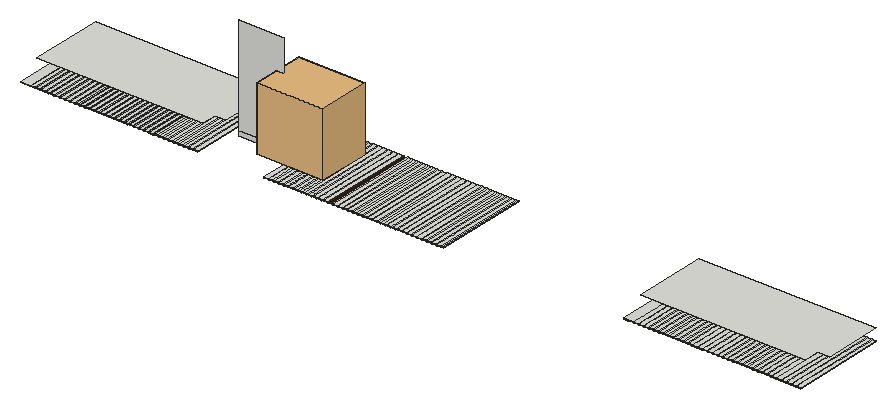
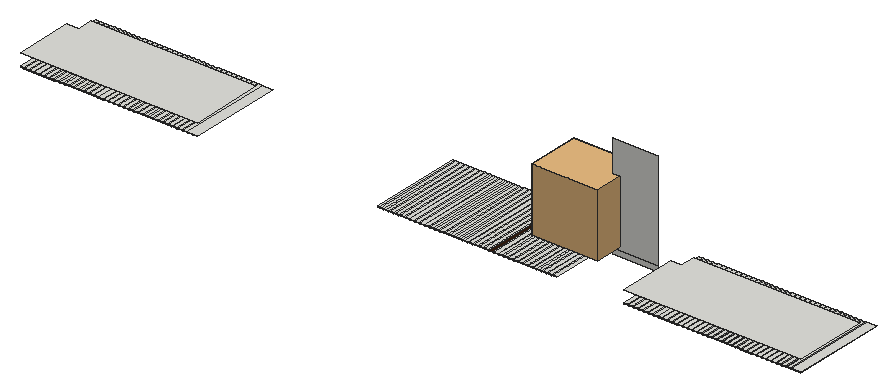
# SketchUp Ruby script. Lengths in inches.
U = 1.inch
M = Sketchup.active_model
def pt(a) = Geom::Point3d.new(a.map { |v| v * U })
def face(e, loops, mat)
  f = e.add_face(loops[0].map { |a| pt(a) })
  loops[1..].each { |l| e.add_face(l.map { |a| pt(a) }).erase! }
  f.material = f.back_material = mat if mat
  f
end
# faces: each face lists its corners as indices into pts; further lists are holes
def faces(e, pts, list, mat = nil) = list.each { |f| face(e, (f[0].is_a?(Array) ? f : [f]).map { |l| l.map { |i| pts[i] } }, mat) }
# xy, xz, yz: faces in a plane at the given z, y or x. An outline is a flat list of corners, or four numbers for a rectangle; further outlines are holes
def ring(l) = l.size == 4 ? [[l[0], l[1]], [l[2], l[1]], [l[2], l[3]], [l[0], l[3]]] : l.each_slice(2).to_a
def flat(e, list, mat, &to3) = list.each { |f| face(e, (f[0].is_a?(Array) ? f : [f]).map { |l| ring(l).map { |u, v| to3.(u, v) } }, mat) }
def xy(e, z, list, mat = nil) = flat(e, list, mat) { |x, y| [x, y, z] }
def xz(e, y, list, mat = nil) = flat(e, list, mat) { |x, z| [x, y, z] }
def yz(e, x, list, mat = nil) = flat(e, list, mat) { |y, z| [x, y, z] }
def lines(e, pts, list) = list.each { |a, b| e.add_line(pt(pts[a]), pt(pts[b])) }
# prism: a flat outline (further loops are holes) pulled along v
def prism(e, loops, v, mat = nil)
  f = face(e, loops, mat); d = Geom::Vector3d.new(v.map { |x| x * U })
  f.pushpull(f.normal.samedirection?(d) ? d.length : -d.length)
end
def box(e, o, s, mat = nil) = prism(e, [[o, [o[0] + s[0], o[1], o[2]], [o[0] + s[0], o[1] + s[1], o[2]], [o[0], o[1] + s[1], o[2]]]], [0, 0, s[2]], mat)
def at(x, y, z, deg = 0) = Geom::Transformation.translation(pt([x, y, z])) * Geom::Transformation.rotation(ORIGIN, Z_AXIS, deg.degrees)
def axes(o, x, y, z) = Geom::Transformation.new([*x, 0, *y, 0, *z, 0, *pt(o).to_a, 1])
def part(name) = M.definitions.add(name)
# library, detail: a bought-in or finely detailed component or shape, given as its bounding box
def library(name, o, s) = part(name).tap { |d| box(d.entities, o, s) }
def detail(e, o, s) = box(e.add_group.entities, o, s)
def put(e, d, t, mat = nil) = e.add_instance(d, t).tap { |i| i.material = mat if mat }
def group(e, t, mat = nil) = e.add_group.tap { |g| g.transformation = t; g.material = mat if mat }.entities
root = M.entities
M.materials.add("[Wood Veneer 01]").color = [51, 28, 15]
c1 = library("Round Planter with Plant",[-35.48,-39.77,0],[80.62,63.55,77.875])
xy(root,253.5625,[[256.68,246.64,261.43,361.27],[262.68,246.64,267.43,361.27],[268.68,246.64,273.43,361.27],[274.68,246.64,279.43,361.27],[280.68,246.64,285.43,361.27],
  [286.68,246.64,291.43,361.27],[292.68,246.64,297.43,361.27],[298.68,246.64,303.43,361.27],[304.68,246.64,309.43,361.27],[310.68,246.64,315.43,361.27],
  [990.25,246.64,995,361.27],[996.25,246.64,1001,361.27],[1002.25,246.64,1007,361.27],[1008.25,246.64,1013,361.27],[1014.25,246.64,1019,361.27],
  [1020.25,246.64,1025,361.27],[1026.25,246.64,1031,361.27],[1032.25,246.64,1037,361.27],[1038.25,246.64,1043,361.27],[1044.25,246.64,1049,361.27]],"[Wood Veneer 01]")
xy(root,253.875,[[244.68,246.64,249.43,361.27],[250.68,246.64,255.43,361.27],[978.25,246.64,983,361.27],[984.25,246.64,989,361.27]],"[Wood Veneer 01]")
xy(root,253.9375,[[100.68,246.64,105.43,361.27],[106.68,246.64,111.43,361.27],[112.68,246.64,117.43,361.27],[118.68,246.64,123.43,361.27],[124.68,246.64,129.43,361.27],
  [130.68,246.64,135.43,361.27],[136.68,246.64,141.43,361.27],[142.68,246.64,147.43,361.27],[148.68,246.64,153.43,361.27],[154.68,246.64,159.43,361.27],
  [160.68,246.64,165.43,361.27],[166.68,246.64,171.43,361.27],[172.68,246.64,177.43,361.27],[178.68,246.64,183.43,361.27],[184.68,246.64,189.43,361.27],
  [190.68,246.64,195.43,361.27],[196.68,246.64,201.43,361.27],[202.68,246.64,207.43,361.27],[208.68,246.64,213.43,361.27],[214.68,246.64,219.43,361.27],
  [220.68,246.64,225.43,361.27],[226.68,246.64,231.43,361.27],[232.68,246.64,237.43,361.27],[238.68,246.64,243.43,361.27],[396.57,246.64,400.96,361.27],
  [402.57,246.64,406.96,361.27],[408.57,246.64,412.96,361.27],[414.57,246.64,418.96,361.27],[420.57,246.64,424.96,361.27],[426.57,246.64,430.96,361.27],
  [432.57,246.64,436.96,361.27],[438.57,246.64,442.96,361.27],[444.57,246.64,448.96,361.27],[450.57,246.64,454.96,361.27],[456.57,246.64,460.96,361.27],
  [462.57,246.64,466.96,361.27],[468.57,246.64,472.96,361.27],[474.57,246.64,478.96,361.27],[480.57,246.64,484.96,361.27],[486.57,246.64,490.96,361.27],
  [492.57,246.64,496.96,361.27],[498.57,246.64,502.96,361.27],[504.57,246.64,508.96,361.27],[510.57,246.64,514.96,361.27],[516.57,246.64,520.96,361.27],
  [522.57,246.64,526.96,361.27],[528.57,246.64,532.96,361.27],[534.57,246.64,538.96,361.27],[540.57,246.64,544.96,361.27],[546.57,246.64,550.96,361.27],
  [552.57,246.64,556.96,361.27],[558.57,246.64,562.96,361.27],[564.57,246.64,568.96,361.27],[570.57,246.64,574.96,361.27],[576.57,246.64,580.96,361.27],
  [582.57,246.64,586.96,361.27],[588.57,246.64,592.96,361.27],[594.57,246.64,598.96,361.27],[600.57,246.64,604.96,361.27],[606.57,246.64,610.96,361.27],
  [612.57,246.64,614.76,361.27],[834.25,246.64,839,361.27],[840.25,246.64,845,361.27],[846.25,246.64,851,361.27],[852.25,246.64,857,361.27],
  [858.25,246.64,863,361.27],[864.25,246.64,869,361.27],[870.25,246.64,875,361.27],[876.25,246.64,881,361.27],[882.25,246.64,887,361.27],
  [888.25,246.64,893,361.27],[894.25,246.64,899,361.27],[900.25,246.64,905,361.27],[906.25,246.64,911,361.27],[912.25,246.64,917,361.27],
  [918.25,246.64,923,361.27],[924.25,246.64,929,361.27],[930.25,246.64,935,361.27],[936.25,246.64,941,361.27],[942.25,246.64,947,361.27],
  [948.25,246.64,953,361.27],[954.25,246.64,959,361.27],[960.25,246.64,965,361.27],[966.25,246.64,971,361.27],[972.25,246.64,977,361.27]],"[Wood Veneer 01]")
xy(root,254.625,[[244.68,246.64,249.43,361.27],[978.25,246.64,983,361.27]])
xy(root,254.6875,[[100.18,246.64,112.68,361.27],[112.68,246.64,117.43,361.27],[117.43,246.64,118.68,361.27],[118.68,246.64,123.43,361.27],[123.43,246.64,124.68,361.27],
  [124.68,246.64,129.43,361.27],[129.43,246.64,130.68,361.27],[130.68,246.64,135.43,361.27],[135.43,246.64,136.68,361.27],[136.68,246.64,141.43,361.27],
  [141.43,246.64,142.68,361.27],[142.68,246.64,147.43,361.27],[147.43,246.64,148.68,361.27],[148.68,246.64,153.43,361.27],[153.43,246.64,154.68,361.27],
  [154.68,246.64,159.43,361.27],[159.43,246.64,160.68,361.27],[160.68,246.64,165.43,361.27],[165.43,246.64,166.68,361.27],[166.68,246.64,171.43,361.27],
  [171.43,246.64,172.68,361.27],[172.68,246.64,177.43,361.27],[177.43,246.64,178.68,361.27],[178.68,246.64,183.43,361.27],[183.43,246.64,184.68,361.27],
  [184.68,246.64,189.43,361.27],[189.43,246.64,190.68,361.27],[190.68,246.64,195.43,361.27],[195.43,246.64,196.68,361.27],[196.68,246.64,201.43,361.27],
  [201.43,246.64,202.68,361.27],[202.68,246.64,207.43,361.27],[207.43,246.64,208.68,361.27],[208.68,246.64,213.43,361.27],[213.43,246.64,214.68,361.27],
  [214.68,246.64,219.43,361.27],[219.43,246.64,220.68,361.27],[220.68,246.64,225.43,361.27],[225.43,246.64,226.68,361.27],[226.68,246.64,231.43,361.27],
  [231.43,246.64,232.68,361.27],[232.68,246.64,237.43,361.27],[237.43,246.64,238.68,361.27],[238.68,246.64,243.43,361.27],[243.43,246.64,244.68,361.27],
  [244.68,246.64,249.43,361.27],[249.43,246.64,250.68,361.27],[250.68,246.64,255.43,361.27],[255.43,246.64,256.68,361.27],[256.68,246.64,261.43,361.27],
  [261.43,246.64,262.68,361.27],[262.68,246.64,267.43,361.27],[267.43,246.64,268.68,361.27],[268.68,246.64,273.43,361.27],[273.43,246.64,274.68,361.27],
  [274.68,246.64,279.43,361.27],[279.43,246.64,280.68,361.27],[280.68,246.64,285.43,361.27],[285.43,246.64,286.68,361.27],[286.68,246.64,291.43,361.27],
  [291.43,246.64,292.68,361.27],[292.68,246.64,297.43,361.27],[297.43,246.64,298.68,361.27],[298.68,246.64,303.43,361.27],[303.43,246.64,304.68,361.27],
  [304.68,246.64,309.43,361.27],[309.43,246.64,310.68,361.27],[310.68,246.64,315.43,361.27],[396.57,246.64,400.96,361.27],[400.96,246.64,402.57,361.27],
  [402.57,246.64,406.96,361.27],[406.96,246.64,408.57,361.27],[408.57,246.64,412.96,361.27],[412.96,246.64,414.57,361.27],[414.57,246.64,418.96,361.27],
  [418.96,246.64,420.57,361.27],[420.57,246.64,424.96,361.27],[424.96,246.64,426.57,361.27],[426.57,246.64,430.96,361.27],[430.96,246.64,432.57,361.27],
  [432.57,246.64,436.96,361.27],[436.96,246.64,438.57,361.27],[438.57,246.64,442.96,361.27],[442.96,246.64,444.57,361.27],[444.57,246.64,448.96,361.27],
  [448.96,246.64,450.57,361.27],[450.57,246.64,454.96,361.27],[454.96,246.64,456.57,361.27],[456.57,246.64,460.96,361.27],[460.96,246.64,462.57,361.27],
  [462.57,246.64,466.96,361.27],[466.96,246.64,468.57,361.27],[468.57,246.64,472.96,361.27],[472.96,246.64,474.57,361.27],[478.96,246.64,480.57,361.27],
  [480.57,246.64,484.96,361.27],[484.96,246.64,486.57,361.27],[486.57,246.64,490.96,361.27],[490.96,246.64,492.57,361.27],[492.57,246.64,496.96,361.27],
  [496.96,246.64,498.57,361.27],[498.57,246.64,502.96,361.27],[502.96,246.64,504.57,361.27],[504.57,246.64,508.96,361.27],[508.96,246.64,510.57,361.27],
  [510.57,246.64,514.96,361.27],[514.96,246.64,516.57,361.27],[516.57,246.64,520.96,361.27],[520.96,246.64,522.57,361.27],[522.57,246.64,526.96,361.27],
  [526.96,246.64,528.57,361.27],[528.57,246.64,532.96,361.27],[532.96,246.64,534.57,361.27],[534.57,246.64,538.96,361.27],[538.96,246.64,540.57,361.27],
  [540.57,246.64,544.96,361.27],[544.96,246.64,546.57,361.27],[546.57,246.64,550.96,361.27],[550.96,246.64,552.57,361.27],[552.57,246.64,556.96,361.27],
  [556.96,246.64,558.57,361.27],[558.57,246.64,562.96,361.27],[562.96,246.64,564.57,361.27],[564.57,246.64,568.96,361.27],[568.96,246.64,570.57,361.27],
  [570.57,246.64,574.96,361.27],[574.96,246.64,576.57,361.27],[576.57,246.64,580.96,361.27],[580.96,246.64,582.57,361.27],[582.57,246.64,586.96,361.27],
  [586.96,246.64,588.57,361.27],[588.57,246.64,592.96,361.27],[592.96,246.64,594.57,361.27],[594.57,246.64,598.96,361.27],[598.96,246.64,600.57,361.27],
  [600.57,246.64,604.96,361.27],[604.96,246.64,606.57,361.27],[606.57,246.64,610.96,361.27],[610.96,246.64,612.57,361.27],[612.57,246.64,614.76,361.27],
  [833.74,246.64,846.25,361.27],[846.25,246.64,851,361.27],[851,246.64,852.25,361.27],[852.25,246.64,857,361.27],[857,246.64,858.25,361.27],
  [858.25,246.64,863,361.27],[863,246.64,864.25,361.27],[864.25,246.64,869,361.27],[869,246.64,870.25,361.27],[870.25,246.64,875,361.27],
  [875,246.64,876.25,361.27],[876.25,246.64,881,361.27],[881,246.64,882.25,361.27],[882.25,246.64,887,361.27],[887,246.64,888.25,361.27],
  [888.25,246.64,893,361.27],[893,246.64,894.25,361.27],[894.25,246.64,899,361.27],[899,246.64,900.25,361.27],[900.25,246.64,905,361.27],
  [905,246.64,906.25,361.27],[906.25,246.64,911,361.27],[911,246.64,912.25,361.27],[912.25,246.64,917,361.27],[917,246.64,918.25,361.27],
  [918.25,246.64,923,361.27],[923,246.64,924.25,361.27],[924.25,246.64,929,361.27],[929,246.64,930.25,361.27],[930.25,246.64,935,361.27],
  [935,246.64,936.25,361.27],[936.25,246.64,941,361.27],[941,246.64,942.25,361.27],[942.25,246.64,947,361.27],[947,246.64,948.25,361.27],
  [948.25,246.64,953,361.27],[953,246.64,954.25,361.27],[954.25,246.64,959,361.27],[959,246.64,960.25,361.27],[960.25,246.64,965,361.27],
  [965,246.64,966.25,361.27],[966.25,246.64,971,361.27],[971,246.64,972.25,361.27],[972.25,246.64,977,361.27],[977,246.64,978.25,361.27],
  [978.25,246.64,983,361.27],[983,246.64,984.25,361.27],[984.25,246.64,989,361.27],[989,246.64,990.25,361.27],[990.25,246.64,995,361.27],
  [995,246.64,996.25,361.27],[996.25,246.64,1001,361.27],[1001,246.64,1002.25,361.27],[1002.25,246.64,1007,361.27],[1007,246.64,1008.25,361.27],
  [1008.25,246.64,1013,361.27],[1013,246.64,1014.25,361.27],[1014.25,246.64,1019,361.27],[1019,246.64,1020.25,361.27],[1020.25,246.64,1025,361.27],
  [1025,246.64,1026.25,361.27],[1026.25,246.64,1031,361.27],[1031,246.64,1032.25,361.27],[1032.25,246.64,1037,361.27],[1037,246.64,1038.25,361.27],
  [1038.25,246.64,1043,361.27],[1043,246.64,1044.25,361.27],[1044.25,246.64,1049,361.27]])
xy(root,269.0625,[[100.18,271.8,301.9,271.8,301.9,290.02,315.43,290.02,315.43,361.27,100.18,361.27],[833.74,271.8,1035.46,271.8,1035.46,290.02,1049,290.02,1049,361.27,833.74,361.27]])
xz(root,293.45,[[328.03,254.6875,382.74,260.6875],[328.03,260.6875,382.74,380.6875]])
yz(root,112.68,[[246.64,253.9375,361.27,254.6875]])
yz(root,118.68,[[246.64,253.9375,361.27,254.6875]])
yz(root,124.68,[[246.64,253.9375,361.27,254.6875]])
yz(root,130.68,[[246.64,253.9375,361.27,254.6875]])
yz(root,136.68,[[246.64,253.9375,361.27,254.6875]])
yz(root,142.68,[[246.64,253.9375,361.27,254.6875]])
yz(root,148.68,[[246.64,253.9375,361.27,254.6875]])
yz(root,154.68,[[246.64,253.9375,361.27,254.6875]])
yz(root,160.68,[[246.64,253.9375,361.27,254.6875]])
yz(root,166.68,[[246.64,253.9375,361.27,254.6875]])
yz(root,172.68,[[246.64,253.9375,361.27,254.6875]])
yz(root,178.68,[[246.64,253.9375,361.27,254.6875]])
yz(root,184.68,[[246.64,253.9375,361.27,254.6875]])
yz(root,190.68,[[246.64,253.9375,361.27,254.6875]])
yz(root,196.68,[[246.64,253.9375,361.27,254.6875]])
yz(root,202.68,[[246.64,253.9375,361.27,254.6875]])
yz(root,208.68,[[246.64,253.9375,361.27,254.6875]])
yz(root,214.68,[[246.64,253.9375,361.27,254.6875]])
yz(root,220.68,[[246.64,253.9375,361.27,254.6875]])
yz(root,226.68,[[246.64,253.9375,361.27,254.6875]])
yz(root,232.68,[[246.64,253.9375,361.27,254.6875]])
yz(root,238.68,[[246.64,253.9375,361.27,254.6875]])
yz(root,244.68,[[246.64,253.875,361.27,254.625],[246.64,254.625,361.27,254.6875]])
yz(root,250.68,[[246.64,253.875,361.27,254.6875]])
yz(root,256.68,[[246.64,253.5625,361.27,254.6875]])
yz(root,262.68,[[246.64,253.5625,361.27,254.6875]])
put(root,c1,at(409.81,303,264.4375))
